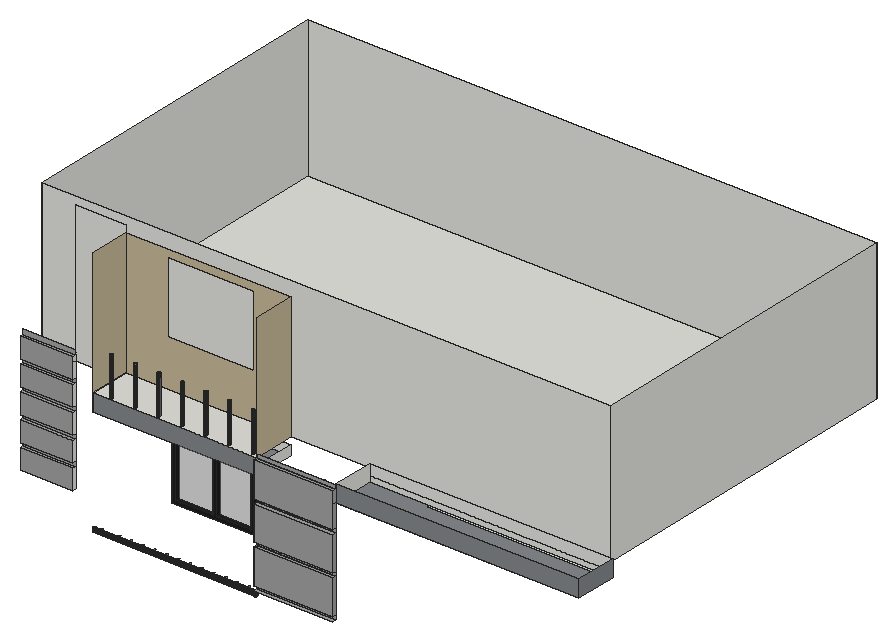
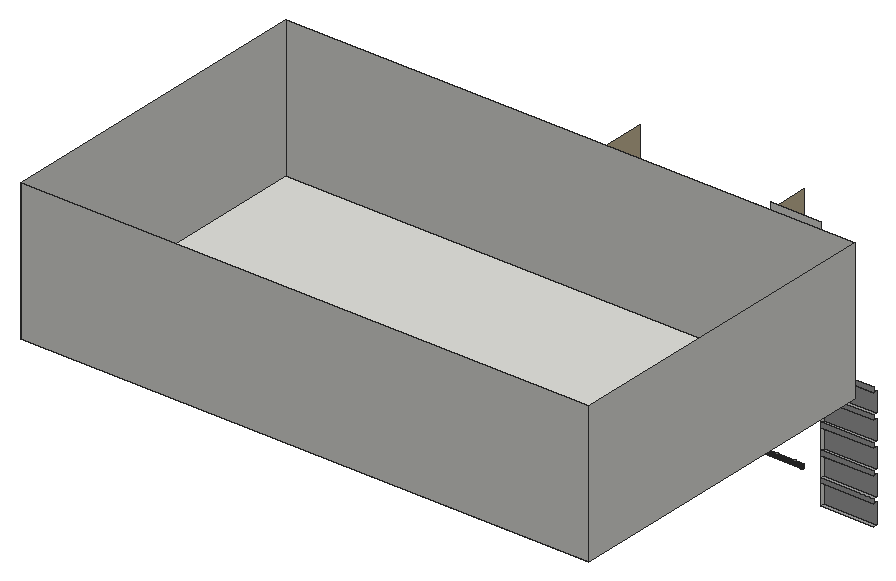
# SketchUp Ruby script. Lengths in inches.
U = 1.inch
M = Sketchup.active_model
def pt(a) = Geom::Point3d.new(a.map { |v| v * U })
def face(e, loops, mat)
  f = e.add_face(loops[0].map { |a| pt(a) })
  loops[1..].each { |l| e.add_face(l.map { |a| pt(a) }).erase! }
  f.material = f.back_material = mat if mat
  f
end
# faces: each face lists its corners as indices into pts; further lists are holes
def faces(e, pts, list, mat = nil) = list.each { |f| face(e, (f[0].is_a?(Array) ? f : [f]).map { |l| l.map { |i| pts[i] } }, mat) }
# xy, xz, yz: faces in a plane at the given z, y or x. An outline is a flat list of corners, or four numbers for a rectangle; further outlines are holes
def ring(l) = l.size == 4 ? [[l[0], l[1]], [l[2], l[1]], [l[2], l[3]], [l[0], l[3]]] : l.each_slice(2).to_a
def flat(e, list, mat, &to3) = list.each { |f| face(e, (f[0].is_a?(Array) ? f : [f]).map { |l| ring(l).map { |u, v| to3.(u, v) } }, mat) }
def xy(e, z, list, mat = nil) = flat(e, list, mat) { |x, y| [x, y, z] }
def xz(e, y, list, mat = nil) = flat(e, list, mat) { |x, z| [x, y, z] }
def yz(e, x, list, mat = nil) = flat(e, list, mat) { |y, z| [x, y, z] }
def lines(e, pts, list) = list.each { |a, b| e.add_line(pt(pts[a]), pt(pts[b])) }
# prism: a flat outline (further loops are holes) pulled along v
def prism(e, loops, v, mat = nil)
  f = face(e, loops, mat); d = Geom::Vector3d.new(v.map { |x| x * U })
  f.pushpull(f.normal.samedirection?(d) ? d.length : -d.length)
end
def box(e, o, s, mat = nil) = prism(e, [[o, [o[0] + s[0], o[1], o[2]], [o[0] + s[0], o[1] + s[1], o[2]], [o[0], o[1] + s[1], o[2]]]], [0, 0, s[2]], mat)
def at(x, y, z, deg = 0) = Geom::Transformation.translation(pt([x, y, z])) * Geom::Transformation.rotation(ORIGIN, Z_AXIS, deg.degrees)
def axes(o, x, y, z) = Geom::Transformation.new([*x, 0, *y, 0, *z, 0, *pt(o).to_a, 1])
def part(name) = M.definitions.add(name)
# library, detail: a bought-in or finely detailed component or shape, given as its bounding box
def library(name, o, s) = part(name).tap { |d| box(d.entities, o, s) }
def detail(e, o, s) = box(e.add_group.entities, o, s)
def put(e, d, t, mat = nil) = e.add_instance(d, t).tap { |i| i.material = mat if mat }
def group(e, t, mat = nil) = e.add_group.tap { |g| g.transformation = t; g.material = mat if mat }.entities
root = M.entities
M.materials.add("[0133_Gray]").color = [128, 128, 128]
M.materials.add("[Blacktop New]").color = [30, 30, 30]
M.materials.add("[Blacktop Old 01]").color = [132, 136, 139]
M.materials.add("[Marble Carrara Gold Floor Tile]").color = [225, 223, 217]
M.materials.add("[Pavers Flagstone Gray]").color = [162, 162, 162]
M.materials.add("[Quartz Light Brown]").color = [199, 184, 152]
M.materials.add("[Translucent Glass Gray]").color = [128, 128, 128]
M.materials["[Translucent Glass Gray]"].alpha = 0.5
xy(root,261.07,[[0,36,45.0625,39]],"[Pavers Flagstone Gray]")
xy(root,263.16,[[95.48,3.83,95.64,3.85,95.79,3.92,95.92,4.02,96.02,4.15,96.08,4.3,96.1,4.46,96.08,4.62,96.02,4.77,95.92,4.9,95.79,5,95.64,5.0625,95.48,5.08,95.32,5.0625,95.17,5,95.04,4.9,94.9375,4.77,94.875,4.62,94.85,4.46,94.875,4.3,94.9375,4.15,95.04,4.02,95.17,3.92,95.32,3.85],[110.48,3.83,110.64,3.85,110.79,3.92,110.92,4.02,111.02,4.15,111.08,4.3,111.1,4.46,111.08,4.62,111.02,4.77,110.92,4.9,110.79,5,110.64,5.0625,110.48,5.08,110.32,5.0625,110.17,5,110.04,4.9,109.9375,4.77,109.875,4.62,109.85,4.46,109.875,4.3,109.9375,4.15,110.04,4.02,110.17,3.92,110.32,3.85],[120.6,3.83,120.77,3.85,120.92,3.92,121.05,4.02,121.15,4.15,121.21,4.3,121.23,4.46,121.21,4.62,121.15,4.77,121.05,4.9,120.92,5,120.77,5.0625,120.6,5.08,120.44,5.0625,120.29,5,120.16,4.9,120.0625,4.77,120,4.62,119.98,4.46,120,4.3,120.0625,4.15,120.16,4.02,120.29,3.92,120.44,3.85],[130.73,3.83,130.89,3.85,131.04,3.92,131.17,4.02,131.27,4.15,131.33,4.3,131.35,4.46,131.33,4.62,131.27,4.77,131.17,4.9,131.04,5,130.89,5.0625,130.73,5.08,130.57,5.0625,130.42,5,130.29,4.9,130.1875,4.77,130.125,4.62,130.1,4.46,130.125,4.3,130.1875,4.15,130.29,4.02,130.42,3.92,130.57,3.85],[140.85,3.83,141.02,3.85,141.17,3.92,141.3,4.02,141.4,4.15,141.46,4.3,141.48,4.46,141.46,4.62,141.4,4.77,141.3,4.9,141.17,5,141.02,5.0625,140.85,5.08,140.69,5.0625,140.54,5,140.41,4.9,140.3125,4.77,140.25,4.62,140.23,4.46,140.25,4.3,140.3125,4.15,140.41,4.02,140.54,3.92,140.69,3.85],
  [150.98,3.83,151.14,3.85,151.29,3.92,151.42,4.02,151.52,4.15,151.58,4.3,151.6,4.46,151.58,4.62,151.52,4.77,151.42,4.9,151.29,5,151.14,5.0625,150.98,5.08,150.82,5.0625,150.67,5,150.54,4.9,150.4375,4.77,150.375,4.62,150.35,4.46,150.375,4.3,150.4375,4.15,150.54,4.02,150.67,3.92,150.82,3.85],[161.1,3.83,161.27,3.85,161.42,3.92,161.55,4.02,161.65,4.15,161.71,4.3,161.73,4.46,161.71,4.62,161.65,4.77,161.55,4.9,161.42,5,161.27,5.0625,161.1,5.08,160.94,5.0625,160.79,5,160.66,4.9,160.5625,4.77,160.5,4.62,160.48,4.46,160.5,4.3,160.5625,4.15,160.66,4.02,160.79,3.92,160.94,3.85],[171.23,3.83,171.39,3.85,171.54,3.92,171.67,4.02,171.77,4.15,171.83,4.3,171.85,4.46,171.83,4.62,171.77,4.77,171.67,4.9,171.54,5,171.39,5.0625,171.23,5.08,171.07,5.0625,170.92,5,170.79,4.9,170.6875,4.77,170.625,4.62,170.6,4.46,170.625,4.3,170.6875,4.15,170.79,4.02,170.92,3.92,171.07,3.85],[181.35,3.83,181.52,3.85,181.67,3.92,181.8,4.02,181.9,4.15,181.96,4.3,181.98,4.46,181.96,4.62,181.9,4.77,181.8,4.9,181.67,5,181.52,5.0625,181.35,5.08,181.19,5.0625,181.04,5,180.91,4.9,180.8125,4.77,180.75,4.62,180.73,4.46,180.75,4.3,180.8125,4.15,180.91,4.02,181.04,3.92,181.19,3.85],[191.48,3.83,191.64,3.85,191.79,3.92,191.92,4.02,192.02,4.15,192.08,4.3,192.1,4.46,192.08,4.62,192.02,4.77,191.92,4.9,191.79,5,191.64,5.0625,191.48,5.08,191.32,5.0625,191.17,5,191.04,4.9,190.9375,4.77,190.875,4.62,190.85,4.46,190.875,4.3,190.9375,4.15,191.04,4.02,191.17,3.92,191.32,3.85],
  [201.6,3.83,201.77,3.85,201.92,3.92,202.05,4.02,202.15,4.15,202.21,4.3,202.23,4.46,202.21,4.62,202.15,4.77,202.05,4.9,201.92,5,201.77,5.0625,201.6,5.08,201.44,5.0625,201.29,5,201.16,4.9,201.0625,4.77,201,4.62,200.98,4.46,201,4.3,201.0625,4.15,201.16,4.02,201.29,3.92,201.44,3.85],[211.73,3.83,211.89,3.85,212.04,3.92,212.17,4.02,212.27,4.15,212.33,4.3,212.35,4.46,212.33,4.62,212.27,4.77,212.17,4.9,212.04,5,211.89,5.0625,211.73,5.08,211.57,5.0625,211.42,5,211.29,4.9,211.1875,4.77,211.125,4.62,211.1,4.46,211.125,4.3,211.1875,4.15,211.29,4.02,211.42,3.92,211.57,3.85],[221.85,3.83,222.02,3.85,222.17,3.92,222.3,4.02,222.4,4.15,222.46,4.3,222.48,4.46,222.46,4.62,222.4,4.77,222.3,4.9,222.17,5,222.02,5.0625,221.85,5.08,221.69,5.0625,221.54,5,221.41,4.9,221.3125,4.77,221.25,4.62,221.23,4.46,221.25,4.3,221.3125,4.15,221.41,4.02,221.54,3.92,221.69,3.85]],"[0133_Gray]")
xy(root,265,[[229.62,0,297.58,3]],"[Pavers Flagstone Gray]")
xy(root,268.62,[[229.62,0,297.58,3]],"[Pavers Flagstone Gray]")
xy(root,278.4375,[[0,36,45.0625,39]],"[Pavers Flagstone Gray]")
xy(root,281.71,[[130.59,36,200.77,39]],"[Blacktop New]")
xy(root,282.51,[[0,36,45.0625,39]],"[Pavers Flagstone Gray]")
xy(root,284.71,[[133.59,36,165.68,39],[168.99,36,197.77,39]],"[Blacktop New]")
xy(root,298.5,[[229.62,0,297.58,3]],"[Pavers Flagstone Gray]")
xy(root,299.875,[[0,36,45.0625,39]],"[Pavers Flagstone Gray]")
xy(root,302.12,[[229.62,0,297.58,3]],"[Pavers Flagstone Gray]")
xy(root,303.95,[[0,36,45.0625,39]],"[Pavers Flagstone Gray]")
xy(root,321.3125,[[0,36,45.0625,39]],"[Pavers Flagstone Gray]")
xy(root,325.39,[[0,36,45.0625,39]],"[Pavers Flagstone Gray]")
xy(root,332,[[229.62,0,297.58,3]],"[Pavers Flagstone Gray]")
xy(root,335.62,[[229.62,0,297.58,3]],"[Pavers Flagstone Gray]")
xy(root,341.28,[[133.59,36,165.68,39],[168.99,36,197.77,39]],"[Blacktop New]")
xy(root,342.75,[[0,36,45.0625,39]],"[Pavers Flagstone Gray]")
xy(root,344.28,[[130.59,36,200.77,39]],"[Blacktop New]")
xy(root,346.82,[[0,36,45.0625,39]],"[Pavers Flagstone Gray]")
xy(root,349.1875,[[355.33,36,420.16,39],[425.68,36,485,39]],"[Blacktop New]")
xy(root,351.5625,[[88.53,3,229.62,39]],"[Blacktop Old 01]")
xy(root,355.1875,[[349.33,36,491,39]])
xy(root,355.1875,[[297.58,3,297.58,39,349.33,39,349.33,36,491,36,491,39,506.625,39,506.625,3]],"[Blacktop Old 01]")
xy(root,360,[[9,48,497.625,333.4375]])
xy(root,364.1875,[[0,36,45.0625,39]],"[Pavers Flagstone Gray]")
xy(root,365.5,[[229.62,0,297.58,3]],"[Pavers Flagstone Gray]")
xy(root,366.04,[[244.21,4.79,244.49,4.8,244.76,4.88,244.99,5.03,245.18,5.23,245.3125,5.48,245.375,5.75,245.36,6.02,245.28,6.29,245.14,6.52,244.93,6.71,244.69,6.84,244.42,6.91,244.14,6.9,243.88,6.82,243.64,6.67,243.45,6.47,243.32,6.22,243.26,5.95,243.27,5.68,243.35,5.41,243.5,5.17,243.7,4.99,243.94,4.85],[264.46,4.79,264.74,4.8,265.01,4.88,265.24,5.03,265.43,5.23,265.5625,5.48,265.625,5.75,265.61,6.02,265.53,6.29,265.39,6.52,265.18,6.71,264.94,6.84,264.67,6.91,264.39,6.9,264.13,6.82,263.89,6.67,263.7,6.47,263.57,6.22,263.51,5.95,263.52,5.68,263.6,5.41,263.75,5.17,263.95,4.99,264.19,4.85],[284.71,4.79,284.99,4.8,285.26,4.88,285.49,5.03,285.68,5.23,285.8125,5.48,285.875,5.75,285.86,6.02,285.78,6.29,285.64,6.52,285.43,6.71,285.19,6.84,284.92,6.91,284.64,6.9,284.38,6.82,284.14,6.67,283.95,6.47,283.82,6.22,283.76,5.95,283.77,5.68,283.85,5.41,284,5.17,284.2,4.99,284.44,4.85],[304.96,4.79,305.24,4.8,305.51,4.88,305.74,5.03,305.93,5.23,306.0625,5.48,306.125,5.75,306.11,6.02,306.03,6.29,305.89,6.52,305.68,6.71,305.44,6.84,305.17,6.91,304.89,6.9,304.63,6.82,304.39,6.67,304.2,6.47,304.07,6.22,304.01,5.95,304.02,5.68,304.1,5.41,304.25,5.17,304.45,4.99,304.69,4.85],[325.21,4.79,325.49,4.8,325.76,4.88,325.99,5.03,326.18,5.23,326.3125,5.48,326.375,5.75,326.36,6.02,326.28,6.29,326.14,6.52,325.93,6.71,325.69,6.84,325.42,6.91,325.14,6.9,324.88,6.82,324.64,6.67,324.45,6.47,324.32,6.22,324.26,5.95,324.27,5.68,324.35,5.41,324.5,5.17,324.7,4.99,324.94,4.85],
  [345.46,4.79,345.74,4.8,346.01,4.88,346.24,5.03,346.43,5.23,346.5625,5.48,346.625,5.75,346.61,6.02,346.53,6.29,346.39,6.52,346.18,6.71,345.94,6.84,345.67,6.91,345.39,6.9,345.13,6.82,344.89,6.67,344.7,6.47,344.57,6.22,344.51,5.95,344.52,5.68,344.6,5.41,344.75,5.17,344.95,4.99,345.19,4.85],[365.71,4.79,365.99,4.8,366.26,4.88,366.49,5.03,366.68,5.23,366.8125,5.48,366.875,5.75,366.86,6.02,366.78,6.29,366.64,6.52,366.43,6.71,366.19,6.84,365.92,6.91,365.64,6.9,365.38,6.82,365.14,6.67,364.95,6.47,364.82,6.22,364.76,5.95,364.77,5.68,364.85,5.41,365,5.17,365.2,4.99,365.44,4.85],[385.96,4.79,386.24,4.8,386.51,4.88,386.74,5.03,386.93,5.23,387.0625,5.48,387.125,5.75,387.11,6.02,387.03,6.29,386.89,6.52,386.68,6.71,386.44,6.84,386.17,6.91,385.89,6.9,385.63,6.82,385.39,6.67,385.2,6.47,385.07,6.22,385.01,5.95,385.02,5.68,385.1,5.41,385.25,5.17,385.45,4.99,385.69,4.85],[406.21,4.79,406.49,4.8,406.76,4.88,406.99,5.03,407.18,5.23,407.3125,5.48,407.375,5.75,407.36,6.02,407.28,6.29,407.14,6.52,406.93,6.71,406.69,6.84,406.42,6.91,406.14,6.9,405.88,6.82,405.64,6.67,405.45,6.47,405.32,6.22,405.26,5.95,405.27,5.68,405.35,5.41,405.5,5.17,405.7,4.99,405.94,4.85]])
xy(root,366.04,[[[88.53,3,229.62,39],[183.46,4.79,183.19,4.85,182.95,4.99,182.75,5.17,182.6,5.41,182.52,5.68,182.51,5.95,182.57,6.22,182.7,6.47,182.89,6.67,183.13,6.82,183.39,6.9,183.67,6.91,183.94,6.84,184.18,6.71,184.39,6.52,184.53,6.29,184.61,6.02,184.625,5.75,184.5625,5.48,184.43,5.23,184.24,5.03,184.01,4.88,183.74,4.8],[203.71,4.79,203.44,4.85,203.2,4.99,203,5.17,202.85,5.41,202.77,5.68,202.76,5.95,202.82,6.22,202.95,6.47,203.14,6.67,203.38,6.82,203.64,6.9,203.92,6.91,204.19,6.84,204.43,6.71,204.64,6.52,204.78,6.29,204.86,6.02,204.875,5.75,204.8125,5.48,204.68,5.23,204.49,5.03,204.26,4.88,203.99,4.8],[223.96,4.79,223.69,4.85,223.45,4.99,223.25,5.17,223.1,5.41,223.02,5.68,223.01,5.95,223.07,6.22,223.2,6.47,223.39,6.67,223.63,6.82,223.89,6.9,224.17,6.91,224.44,6.84,224.68,6.71,224.89,6.52,225.03,6.29,225.11,6.02,225.125,5.75,225.0625,5.48,224.93,5.23,224.74,5.03,224.51,4.88,224.24,4.8],[102.46,4.79,102.19,4.85,101.95,4.99,101.75,5.17,101.6,5.41,101.52,5.68,101.51,5.95,101.57,6.22,101.7,6.47,101.89,6.67,102.13,6.82,102.39,6.9,102.67,6.91,102.94,6.84,103.18,6.71,103.39,6.52,103.53,6.29,103.61,6.02,103.625,5.75,103.5625,5.48,103.43,5.23,103.24,5.03,103.01,4.88,102.74,4.8],[122.71,4.79,122.44,4.85,122.2,4.99,122,5.17,121.85,5.41,121.77,5.68,121.76,5.95,121.82,6.22,121.95,6.47,122.14,6.67,122.38,6.82,122.64,6.9,122.92,6.91,123.19,6.84,123.43,6.71,123.64,6.52,123.78,6.29,123.86,6.02,123.875,5.75,123.8125,5.48,123.68,5.23,123.49,5.03,123.26,4.88,122.99,4.8],[142.96,4.79,142.69,4.85,142.45,4.99,142.25,5.17,142.1,5.41,142.02,5.68,142.01,5.95,142.07,6.22,142.2,6.47,142.39,6.67,142.63,6.82,142.89,6.9,143.17,6.91,143.44,6.84,143.68,6.71,143.89,6.52,144.03,6.29,144.11,6.02,144.125,5.75,144.0625,5.48,143.93,5.23,143.74,5.03,143.51,4.88,143.24,4.8],[163.21,4.79,162.94,4.85,162.7,4.99,162.5,5.17,162.35,5.41,162.27,5.68,162.26,5.95,162.32,6.22,162.45,6.47,162.64,6.67,162.88,6.82,163.14,6.9,163.42,6.91,163.69,6.84,163.93,6.71,164.14,6.52,164.28,6.29,164.36,6.02,164.375,5.75,164.3125,5.48,164.18,5.23,163.99,5.03,163.76,4.88,163.49,4.8]]],"[Marble Carrara Gold Floor Tile]")
xz(root,0,[[229.62,268.62,297.58,298.5],[229.62,302.12,297.58,332],[229.62,335.62,297.58,365.5]],"[Pavers Flagstone Gray]")
xz(root,3,[[229.62,268.62,297.58,298.5],[229.62,302.12,297.58,332],[229.62,335.62,297.58,365.5]])
xz(root,3,[[88.53,351.5625,229.62,366.04],[297.58,355.1875,506.625,369.51]],"[Blacktop Old 01]")
xz(root,3,[[229.62,265,297.58,268.62],[229.62,298.5,297.58,302.12],[229.62,332,297.58,335.62],[229.62,365.5,297.58,369.12]],"[Pavers Flagstone Gray]")
xz(root,36,[[[130.59,281.71,200.77,344.28],[133.59,284.71,165.68,341.28],[168.99,284.71,197.77,341.28]]],"[Blacktop New]")
xz(root,36,[[0,261.07,45.0625,278.4375],[0,282.51,45.0625,299.875],[0,303.95,45.0625,321.3125],[0,325.39,45.0625,342.75],[0,346.82,45.0625,364.1875]],"[Pavers Flagstone Gray]")
xz(root,39,[[88.53,351.5625,229.62,359.8125],[297.58,355.1875,506.625,359.8125],[88.53,359.8125,229.62,360],[297.58,359.8125,506.625,369.51],[45.0625,360,88.53,480]])
xz(root,39,[[0,278.4375,45.0625,282.51],[0,299.875,45.0625,303.95],[0,321.3125,45.0625,325.39],[0,342.75,45.0625,346.82],[0,364.1875,45.0625,368.26]],"[Pavers Flagstone Gray]")
xz(root,39,[[[88.53,366.04,229.62,473.6875],[124.42,405.86,198.67,467.74]]],"[Quartz Light Brown]")
xz(root,39,[[133.59,284.71,165.68,341.28],[168.99,284.71,197.77,341.28]],"[Translucent Glass Gray]")
xz(root,48,[[9,360,497.625,480]])
xz(root,333.4375,[[9,360,497.625,480]])
yz(root,9,[[48,360,333.4375,480]])
yz(root,45.0625,[[36,261.07,39,278.4375],[36,282.51,39,299.875],[36,303.95,39,321.3125],[36,325.39,39,342.75],[36,346.82,39,360],
  [36,360,39,364.1875]])
yz(root,88.53,[[3,351.5625,39,360],[3,360,39,366.04]])
yz(root,88.53,[[[3,366.04,39,473.6875],[3.75,370.61,3.57,370.63,3.41,370.7,3.27,370.81,3.16,370.95,3.09,371.11,3.06,371.29,3.09,371.47,3.16,371.64,3.27,371.78,3.41,371.89,3.57,371.96,3.75,371.98,3.93,371.96,4.1,371.89,4.24,371.78,4.35,371.64,4.42,371.47,4.44,371.29,4.42,371.11,4.35,370.95,4.24,370.81,4.1,370.7,3.93,370.63],[3.75,374.36,3.57,374.38,3.41,374.45,3.27,374.56,3.16,374.7,3.09,374.86,3.06,375.04,3.09,375.22,3.16,375.39,3.27,375.53,3.41,375.64,3.57,375.71,3.75,375.73,3.93,375.71,4.1,375.64,4.24,375.53,4.35,375.39,4.42,375.22,4.44,375.04,4.42,374.86,4.35,374.7,4.24,374.56,4.1,374.45,3.93,374.38],[3.75,378.11,3.57,378.13,3.41,378.2,3.27,378.31,3.16,378.45,3.09,378.61,3.06,378.79,3.09,378.97,3.16,379.14,3.27,379.28,3.41,379.39,3.57,379.46,3.75,379.48,3.93,379.46,4.1,379.39,4.24,379.28,4.35,379.14,4.42,378.97,4.44,378.79,4.42,378.61,4.35,378.45,4.24,378.31,4.1,378.2,3.93,378.13],[3.75,381.86,3.57,381.88,3.41,381.95,3.27,382.06,3.16,382.2,3.09,382.36,3.06,382.54,3.09,382.72,3.16,382.89,3.27,383.03,3.41,383.14,3.57,383.21,3.75,383.23,3.93,383.21,4.1,383.14,4.24,383.03,4.35,382.89,4.42,382.72,4.44,382.54,4.42,382.36,4.35,382.2,4.24,382.06,4.1,381.95,3.93,381.88],[3.75,385.61,3.57,385.63,3.41,385.7,3.27,385.81,3.16,385.95,3.09,386.11,3.06,386.29,3.09,386.47,3.16,386.64,3.27,386.78,3.41,386.89,3.57,386.96,3.75,386.98,3.93,386.96,4.1,386.89,4.24,386.78,4.35,386.64,4.42,386.47,4.44,386.29,4.42,386.11,4.35,385.95,4.24,385.81,4.1,385.7,3.93,385.63],[3.75,389.36,3.57,389.38,3.41,389.45,3.27,389.56,3.16,389.7,3.09,389.86,3.06,390.04,3.09,390.22,3.16,390.39,3.27,390.53,3.41,390.64,3.57,390.71,3.75,390.73,3.93,390.71,4.1,390.64,4.24,390.53,4.35,390.39,4.42,390.22,4.44,390.04,4.42,389.86,4.35,389.7,4.24,389.56,4.1,389.45,3.93,389.38],[3.75,393.11,3.57,393.13,3.41,393.2,3.27,393.31,3.16,393.45,3.09,393.61,3.06,393.79,3.09,393.97,3.16,394.14,3.27,394.28,3.41,394.39,3.57,394.46,3.75,394.48,3.93,394.46,4.1,394.39,4.24,394.28,4.35,394.14,4.42,393.97,4.44,393.79,4.42,393.61,4.35,393.45,4.24,393.31,4.1,393.2,3.93,393.13],[3.75,396.86,3.57,396.88,3.41,396.95,3.27,397.06,3.16,397.2,3.09,397.36,3.06,397.54,3.09,397.72,3.16,397.89,3.27,398.03,3.41,398.14,3.57,398.21,3.75,398.23,3.93,398.21,4.1,398.14,4.24,398.03,4.35,397.89,4.42,397.72,4.44,397.54,4.42,397.36,4.35,397.2,4.24,397.06,4.1,396.95,3.93,396.88]]],"[Quartz Light Brown]")
yz(root,130.59,[[36,281.71,39,344.28]],"[Blacktop New]")
yz(root,133.59,[[36,284.71,39,341.28]],"[Blacktop New]")
yz(root,165.68,[[36,284.71,39,341.28]],"[Blacktop New]")
yz(root,168.99,[[36,284.71,39,341.28]],"[Blacktop New]")
yz(root,197.77,[[36,284.71,39,341.28]],"[Blacktop New]")
yz(root,200.77,[[36,281.71,39,344.28]],"[Blacktop New]")
yz(root,229.62,[[3,351.5625,39,360]])
yz(root,229.62,[[0,268.62,3,298.5],[0,302.12,3,332],[0,335.62,3,365.5]],"[Pavers Flagstone Gray]")
yz(root,229.62,[[[3,366.04,39,473.6875],[3.75,389.36,3.93,389.38,4.1,389.45,4.24,389.56,4.35,389.7,4.42,389.86,4.44,390.04,4.42,390.22,4.35,390.39,4.24,390.53,4.1,390.64,3.93,390.71,3.75,390.73,3.57,390.71,3.41,390.64,3.27,390.53,3.16,390.39,3.09,390.22,3.06,390.04,3.09,389.86,3.16,389.7,3.27,389.56,3.41,389.45,3.57,389.38],[3.75,385.61,3.93,385.63,4.1,385.7,4.24,385.81,4.35,385.95,4.42,386.11,4.44,386.29,4.42,386.47,4.35,386.64,4.24,386.78,4.1,386.89,3.93,386.96,3.75,386.98,3.57,386.96,3.41,386.89,3.27,386.78,3.16,386.64,3.09,386.47,3.06,386.29,3.09,386.11,3.16,385.95,3.27,385.81,3.41,385.7,3.57,385.63],[3.75,381.86,3.93,381.88,4.1,381.95,4.24,382.06,4.35,382.2,4.42,382.36,4.44,382.54,4.42,382.72,4.35,382.89,4.24,383.03,4.1,383.14,3.93,383.21,3.75,383.23,3.57,383.21,3.41,383.14,3.27,383.03,3.16,382.89,3.09,382.72,3.06,382.54,3.09,382.36,3.16,382.2,3.27,382.06,3.41,381.95,3.57,381.88],[3.75,378.11,3.93,378.13,4.1,378.2,4.24,378.31,4.35,378.45,4.42,378.61,4.44,378.79,4.42,378.97,4.35,379.14,4.24,379.28,4.1,379.39,3.93,379.46,3.75,379.48,3.57,379.46,3.41,379.39,3.27,379.28,3.16,379.14,3.09,378.97,3.06,378.79,3.09,378.61,3.16,378.45,3.27,378.31,3.41,378.2,3.57,378.13]]],"[Quartz Light Brown]")
yz(root,297.58,[[3,355.1875,39,369.51]])
yz(root,297.58,[[0,268.62,3,298.5],[0,302.12,3,332],[0,335.62,3,355.1875],[0,355.1875,3,365.5]],"[Pavers Flagstone Gray]")
yz(root,497.625,[[48,360,333.4375,480]])
yz(root,506.625,[[3,355.1875,39,369.51]],"[Blacktop Old 01]")
p = [[88.53,3.34,258.9375],[88.53,3.43,258.9],[229.62,3.43,258.9],[229.62,3.34,258.9375],[88.53,3.26,259],[229.62,3.26,259],
  [88.53,3.53,258.89],[229.62,3.53,258.89],[88.53,3.625,258.9],[229.62,3.625,258.9],[88.53,3.71,258.9375],[229.62,3.71,258.9375],
  [88.53,3.79,259],[229.62,3.79,259],[88.53,3.2,259.08],[229.62,3.2,259.08],[88.53,3.85,259.08],[229.62,3.85,259.08],
  [88.53,3.16,259.17],[229.62,3.16,259.17],[88.53,3.89,259.17],[229.62,3.89,259.17],[88.53,3.15,259.26],[229.62,3.15,259.26],
  [88.53,3.9,259.26],[229.62,3.9,259.26],[88.53,3.16,259.36],[229.62,3.16,259.36],[88.53,3.89,259.36],[229.62,3.89,259.36],
  [88.53,3.2,259.45],[229.62,3.2,259.45],[88.53,3.85,259.45],[229.62,3.85,259.45],[88.53,3.26,259.53],[229.62,3.26,259.53],
  [88.53,3.34,259.59],[229.62,3.34,259.59],[88.53,3.79,259.53],[88.53,3.71,259.59],[229.62,3.71,259.59],[229.62,3.79,259.53],
  [88.53,3.43,259.625],[229.62,3.43,259.625],[88.53,3.53,259.64],[229.62,3.53,259.64],[88.53,3.625,259.625],[229.62,3.625,259.625],
  [88.53,3.34,260.5],[88.53,3.43,260.46],[229.62,3.43,260.46],[229.62,3.34,260.5],[88.53,3.26,260.56],[229.62,3.26,260.56],
  [88.53,3.53,260.45],[229.62,3.53,260.45],[88.53,3.625,260.46],[229.62,3.625,260.46],[88.53,3.71,260.5],[229.62,3.71,260.5],
  [88.53,3.79,260.56],[229.62,3.79,260.56],[88.53,3.2,260.64],[229.62,3.2,260.64],[88.53,3.16,260.73],[229.62,3.16,260.73],
  [88.53,3.85,260.64],[229.62,3.85,260.64],[88.53,3.89,260.73],[229.62,3.89,260.73],[88.53,3.15,260.83],[229.62,3.15,260.83],
  [88.53,3.9,260.83],[229.62,3.9,260.83],[88.53,3.16,260.92],[229.62,3.16,260.92],[88.53,3.89,260.92],[229.62,3.89,260.92],
  [88.53,3.2,261.01],[229.62,3.2,261.01],[88.53,3.85,261.01],[229.62,3.85,261.01],[88.53,3.26,261.09],[229.62,3.26,261.09],
  [88.53,3.79,261.09],[229.62,3.79,261.09],[88.53,3.34,261.15],[229.62,3.34,261.15],[88.53,3.43,261.1875],[229.62,3.43,261.1875],
  [88.53,3.71,261.15],[88.53,3.625,261.1875],[229.62,3.625,261.1875],[229.62,3.71,261.15],[88.53,3.53,261.2],[229.62,3.53,261.2],
  [88.53,3.34,262.0625],[88.53,3.43,262.03],[229.62,3.43,262.03],[229.62,3.34,262.0625],[88.53,3.53,262.01],[229.62,3.53,262.01],
  [88.53,3.625,262.03],[229.62,3.625,262.03],[88.53,3.71,262.0625],[229.62,3.71,262.0625],[88.53,3.2,262.2],[88.53,3.26,262.12],
  [229.62,3.26,262.12],[229.62,3.2,262.2],[88.53,3.79,262.12],[229.62,3.79,262.12],[88.53,3.85,262.2],[229.62,3.85,262.2],
  [88.53,3.16,262.29],[229.62,3.16,262.29],[88.53,3.89,262.29],[229.62,3.89,262.29],[88.53,3.15,262.39],[229.62,3.15,262.39],
  [88.53,3.9,262.39],[229.62,3.9,262.39],[88.53,3.16,262.48],[229.62,3.16,262.48],[88.53,3.89,262.48],[229.62,3.89,262.48],
  [88.53,3.2,262.58],[229.62,3.2,262.58],[88.53,3.85,262.58],[229.62,3.85,262.58],[88.53,3.26,262.65],[229.62,3.26,262.65],
  [88.53,3.79,262.65],[229.62,3.79,262.65],[88.53,3.34,262.71],[229.62,3.34,262.71],[88.53,3.43,262.75],[229.62,3.43,262.75],
  [88.53,3.53,262.76],[229.62,3.53,262.76],[88.53,3.625,262.75],[229.62,3.625,262.75],[88.53,3.71,262.71],[229.62,3.71,262.71],
  [102.19,4.85,366.04],[102.46,4.79,366.04],[102.46,4.79,399.54],[102.19,4.85,399.54],[102.74,4.8,366.04],[102.74,4.8,399.54],
  [103.01,4.88,366.04],[103.01,4.88,399.54],[122.44,4.85,366.04],[122.71,4.79,366.04],[122.71,4.79,399.54],[122.44,4.85,399.54],
  [122.99,4.8,366.04],[122.99,4.8,399.54],[123.26,4.88,366.04],[123.26,4.88,399.54],[142.69,4.85,366.04],[142.96,4.79,366.04],
  [142.96,4.79,399.54],[142.69,4.85,399.54],[143.24,4.8,366.04],[143.24,4.8,399.54],[143.51,4.88,366.04],[143.51,4.88,399.54],
  [162.94,4.85,366.04],[163.21,4.79,366.04],[163.21,4.79,399.54],[162.94,4.85,399.54],[163.49,4.8,366.04],[163.49,4.8,399.54],
  [163.76,4.88,366.04],[163.76,4.88,399.54],[183.19,4.85,366.04],[183.46,4.79,366.04],[183.46,4.79,399.54],[183.19,4.85,399.54],
  [183.74,4.8,366.04],[183.74,4.8,399.54],[184.01,4.88,366.04],[184.01,4.88,399.54],[203.44,4.85,366.04],[203.71,4.79,366.04],
  [203.71,4.79,399.54],[203.44,4.85,399.54],[203.99,4.8,366.04],[203.99,4.8,399.54],[204.26,4.88,366.04],[204.26,4.88,399.54],
  [223.69,4.85,366.04],[223.96,4.79,366.04],[223.96,4.79,399.54],[223.69,4.85,399.54],[224.24,4.8,366.04],[224.24,4.8,399.54],
  [224.51,4.88,366.04],[224.51,4.88,399.54],[101.95,4.99,366.04],[101.95,4.99,399.54],[103.24,5.03,366.04],[103.24,5.03,399.54],
  [122.2,4.99,366.04],[122.2,4.99,399.54],[123.49,5.03,366.04],[123.49,5.03,399.54],[142.45,4.99,366.04],[142.45,4.99,399.54],
  [143.74,5.03,366.04],[143.74,5.03,399.54],[162.7,4.99,366.04],[162.7,4.99,399.54],[163.99,5.03,366.04],[163.99,5.03,399.54],
  [182.95,4.99,366.04],[182.95,4.99,399.54],[184.24,5.03,366.04],[184.24,5.03,399.54],[203.2,4.99,366.04],[203.2,4.99,399.54],
  [204.49,5.03,366.04],[204.49,5.03,399.54],[223.45,4.99,366.04],[223.45,4.99,399.54],[224.74,5.03,366.04],[224.74,5.03,399.54],
  [101.75,5.17,366.04],[101.75,5.17,399.54],[103.43,5.23,366.04],[103.43,5.23,399.54],[122,5.17,366.04],[122,5.17,399.54],
  [123.68,5.23,366.04],[123.68,5.23,399.54],[142.25,5.17,366.04],[142.25,5.17,399.54],[143.93,5.23,366.04],[143.93,5.23,399.54],
  [162.5,5.17,366.04],[162.5,5.17,399.54],[164.18,5.23,366.04],[164.18,5.23,399.54],[182.75,5.17,366.04],[182.75,5.17,399.54],
  [184.43,5.23,366.04],[184.43,5.23,399.54],[203,5.17,366.04],[203,5.17,399.54],[204.68,5.23,366.04],[204.68,5.23,399.54],
  [223.25,5.17,366.04],[223.25,5.17,399.54],[224.93,5.23,366.04],[224.93,5.23,399.54],[101.6,5.41,366.04],[101.6,5.41,399.54],
  [103.5625,5.48,366.04],[103.5625,5.48,399.54],[121.85,5.41,366.04],[121.85,5.41,399.54],[123.8125,5.48,366.04],[123.8125,5.48,399.54],
  [142.1,5.41,366.04],[142.1,5.41,399.54],[144.0625,5.48,366.04],[144.0625,5.48,399.54],[162.35,5.41,366.04],[162.35,5.41,399.54],
  [164.3125,5.48,366.04],[164.3125,5.48,399.54],[182.6,5.41,366.04],[182.6,5.41,399.54],[184.5625,5.48,366.04],[184.5625,5.48,399.54],
  [202.85,5.41,366.04],[202.85,5.41,399.54],[204.8125,5.48,366.04],[204.8125,5.48,399.54],[223.1,5.41,366.04],[223.1,5.41,399.54],
  [225.0625,5.48,366.04],[225.0625,5.48,399.54],[101.52,5.68,366.04],[101.52,5.68,399.54],[121.77,5.68,366.04],[121.77,5.68,399.54],
  [142.02,5.68,366.04],[142.02,5.68,399.54],[162.27,5.68,366.04],[162.27,5.68,399.54],[182.52,5.68,366.04],[182.52,5.68,399.54],
  [202.77,5.68,366.04],[202.77,5.68,399.54],[223.02,5.68,366.04],[223.02,5.68,399.54],[103.625,5.75,366.04],[103.625,5.75,399.54],
  [123.875,5.75,366.04],[123.875,5.75,399.54],[144.125,5.75,366.04],[144.125,5.75,399.54],[164.375,5.75,366.04],[164.375,5.75,399.54],
  [184.625,5.75,366.04],[184.625,5.75,399.54],[204.875,5.75,366.04],[204.875,5.75,399.54],[225.125,5.75,366.04],[225.125,5.75,399.54],
  [101.51,5.95,366.04],[101.51,5.95,399.54],[103.61,6.02,366.04],[103.61,6.02,399.54],[121.76,5.95,366.04],[121.76,5.95,399.54],
  [123.86,6.02,366.04],[123.86,6.02,399.54],[142.01,5.95,366.04],[142.01,5.95,399.54],[144.11,6.02,366.04],[144.11,6.02,399.54],
  [162.26,5.95,366.04],[162.26,5.95,399.54],[164.36,6.02,366.04],[164.36,6.02,399.54],[182.51,5.95,366.04],[182.51,5.95,399.54],
  [184.61,6.02,366.04],[184.61,6.02,399.54],[202.76,5.95,366.04],[202.76,5.95,399.54],[204.86,6.02,366.04],[204.86,6.02,399.54],
  [223.01,5.95,366.04],[223.01,5.95,399.54],[225.11,6.02,366.04],[225.11,6.02,399.54],[101.57,6.22,366.04],[101.57,6.22,399.54],
  [103.53,6.29,366.04],[103.53,6.29,399.54],[121.82,6.22,366.04],[121.82,6.22,399.54],[123.78,6.29,366.04],[123.78,6.29,399.54],
  [142.07,6.22,366.04],[142.07,6.22,399.54],[144.03,6.29,366.04],[144.03,6.29,399.54],[162.32,6.22,366.04],[162.32,6.22,399.54],
  [164.28,6.29,366.04],[164.28,6.29,399.54],[182.57,6.22,366.04],[182.57,6.22,399.54],[184.53,6.29,366.04],[184.53,6.29,399.54],
  [202.82,6.22,366.04],[202.82,6.22,399.54],[204.78,6.29,366.04],[204.78,6.29,399.54],[223.07,6.22,366.04],[223.07,6.22,399.54],
  [225.03,6.29,366.04],[225.03,6.29,399.54],[101.7,6.47,366.04],[101.7,6.47,399.54],[121.95,6.47,366.04],[121.95,6.47,399.54],
  [142.2,6.47,366.04],[142.2,6.47,399.54],[162.45,6.47,366.04],[162.45,6.47,399.54],[182.7,6.47,366.04],[182.7,6.47,399.54],
  [202.95,6.47,366.04],[202.95,6.47,399.54],[223.2,6.47,366.04],[223.2,6.47,399.54],[103.39,6.52,366.04],[103.39,6.52,399.54],
  [123.64,6.52,366.04],[123.64,6.52,399.54],[143.89,6.52,366.04],[143.89,6.52,399.54],[164.14,6.52,366.04],[164.14,6.52,399.54],
  [184.39,6.52,366.04],[184.39,6.52,399.54],[204.64,6.52,366.04],[204.64,6.52,399.54],[224.89,6.52,366.04],[224.89,6.52,399.54],
  [101.89,6.67,366.04],[101.89,6.67,399.54],[103.18,6.71,366.04],[103.18,6.71,399.54],[122.14,6.67,366.04],[122.14,6.67,399.54],
  [123.43,6.71,366.04],[123.43,6.71,399.54],[142.39,6.67,366.04],[142.39,6.67,399.54],[143.68,6.71,366.04],[143.68,6.71,399.54],
  [162.64,6.67,366.04],[162.64,6.67,399.54],[163.93,6.71,366.04],[163.93,6.71,399.54],[182.89,6.67,366.04],[182.89,6.67,399.54],
  [184.18,6.71,366.04],[184.18,6.71,399.54],[203.14,6.67,366.04],[203.14,6.67,399.54],[204.43,6.71,366.04],[204.43,6.71,399.54],
  [223.39,6.67,366.04],[223.39,6.67,399.54],[224.68,6.71,366.04],[224.68,6.71,399.54],[102.13,6.82,366.04],[102.13,6.82,399.54],
  [102.94,6.84,366.04],[102.94,6.84,399.54],[122.38,6.82,366.04],[122.38,6.82,399.54],[123.19,6.84,366.04],[123.19,6.84,399.54],
  [142.63,6.82,366.04],[142.63,6.82,399.54],[143.44,6.84,366.04],[143.44,6.84,399.54],[162.88,6.82,366.04],[162.88,6.82,399.54],
  [163.69,6.84,366.04],[163.69,6.84,399.54],[183.13,6.82,366.04],[183.13,6.82,399.54],[183.94,6.84,366.04],[183.94,6.84,399.54],
  [203.38,6.82,366.04],[203.38,6.82,399.54],[204.19,6.84,366.04],[204.19,6.84,399.54],[223.63,6.82,366.04],[223.63,6.82,399.54],
  [224.44,6.84,366.04],[224.44,6.84,399.54],[102.39,6.9,366.04],[102.39,6.9,399.54],[102.67,6.91,366.04],[102.67,6.91,399.54],
  [122.64,6.9,366.04],[122.64,6.9,399.54],[122.92,6.91,366.04],[122.92,6.91,399.54],[142.89,6.9,366.04],[142.89,6.9,399.54],
  [143.17,6.91,366.04],[143.17,6.91,399.54],[163.14,6.9,366.04],[163.14,6.9,399.54],[163.42,6.91,366.04],[163.42,6.91,399.54],
  [183.39,6.9,366.04],[183.39,6.9,399.54],[183.67,6.91,366.04],[183.67,6.91,399.54],[203.64,6.9,366.04],[203.64,6.9,399.54],
  [203.92,6.91,366.04],[203.92,6.91,399.54],[223.89,6.9,366.04],[223.89,6.9,399.54],[224.17,6.91,366.04],[224.17,6.91,399.54]]
faces(root,p,[[0,1,2,3],[4,0,3,5],[1,6,7,2],[6,8,9,7],[8,10,11,9],[10,12,13,11],[14,4,5,15],[12,16,17,13],
  [18,14,15,19],[16,20,21,17],[22,18,19,23],[20,24,25,21],[26,22,23,27],[24,28,29,25],[30,26,27,31],[28,32,33,29],
  [34,30,31,35],[36,34,35,37],[38,39,40,41],[32,38,41,33],[42,36,37,43],[44,42,43,45],[46,44,45,47],[39,46,47,40],
  [48,49,50,51],[52,48,51,53],[49,54,55,50],[54,56,57,55],[56,58,59,57],[58,60,61,59],[62,52,53,63],[64,62,63,65],
  [60,66,67,61],[66,68,69,67],[70,64,65,71],[68,72,73,69],[74,70,71,75],[72,76,77,73],[78,74,75,79],[76,80,81,77],
  [82,78,79,83],[80,84,85,81],[86,82,83,87],[88,86,87,89],[90,91,92,93],[84,90,93,85],[94,88,89,95],[91,94,95,92],
  [96,97,98,99],[97,100,101,98],[100,102,103,101],[102,104,105,103],[106,107,108,109],[107,96,99,108],[104,110,111,105],[110,112,113,111],
  [114,106,109,115],[112,116,117,113],[118,114,115,119],[116,120,121,117],[122,118,119,123],[120,124,125,121],[126,122,123,127],[124,128,129,125],
  [130,126,127,131],[128,132,133,129],[134,130,131,135],[136,134,135,137],[138,136,137,139],[140,138,139,141],[142,140,141,143],[132,142,143,133],
  [144,145,146,147],[145,148,149,146],[148,150,151,149],[152,153,154,155],[153,156,157,154],[156,158,159,157],[160,161,162,163],[161,164,165,162],
  [164,166,167,165],[168,169,170,171],[169,172,173,170],[172,174,175,173],[176,177,178,179],[177,180,181,178],[180,182,183,181],[184,185,186,187],
  [185,188,189,186],[188,190,191,189],[192,193,194,195],[193,196,197,194],[196,198,199,197],[200,144,147,201],[150,202,203,151],[204,152,155,205],
  [158,206,207,159],[208,160,163,209],[166,210,211,167],[212,168,171,213],[174,214,215,175],[216,176,179,217],[182,218,219,183],[220,184,187,221],
  [190,222,223,191],[224,192,195,225],[198,226,227,199],[228,200,201,229],[202,230,231,203],[232,204,205,233],[206,234,235,207],[236,208,209,237],
  [210,238,239,211],[240,212,213,241],[214,242,243,215],[244,216,217,245],[218,246,247,219],[248,220,221,249],[222,250,251,223],[252,224,225,253],
  [226,254,255,227],[256,228,229,257],[230,258,259,231],[260,232,233,261],[234,262,263,235],[264,236,237,265],[238,266,267,239],[268,240,241,269],
  [242,270,271,243],[272,244,245,273],[246,274,275,247],[276,248,249,277],[250,278,279,251],[280,252,253,281],[254,282,283,255],[284,256,257,285],
  [286,260,261,287],[288,264,265,289],[290,268,269,291],[292,272,273,293],[294,276,277,295],[296,280,281,297],[258,298,299,259],[262,300,301,263],
  [266,302,303,267],[270,304,305,271],[274,306,307,275],[278,308,309,279],[282,310,311,283],[312,284,285,313],[298,314,315,299],[316,286,287,317],
  [300,318,319,301],[320,288,289,321],[302,322,323,303],[324,290,291,325],[304,326,327,305],[328,292,293,329],[306,330,331,307],[332,294,295,333],
  [308,334,335,309],[336,296,297,337],[310,338,339,311],[340,312,313,341],[314,342,343,315],[344,316,317,345],[318,346,347,319],[348,320,321,349],
  [322,350,351,323],[352,324,325,353],[326,354,355,327],[356,328,329,357],[330,358,359,331],[360,332,333,361],[334,362,363,335],[364,336,337,365],
  [338,366,367,339],[368,340,341,369],[370,344,345,371],[372,348,349,373],[374,352,353,375],[376,356,357,377],[378,360,361,379],[380,364,365,381],
  [342,382,383,343],[346,384,385,347],[350,386,387,351],[354,388,389,355],[358,390,391,359],[362,392,393,363],[366,394,395,367],[396,368,369,397],
  [382,398,399,383],[400,370,371,401],[384,402,403,385],[404,372,373,405],[386,406,407,387],[408,374,375,409],[388,410,411,389],[412,376,377,413],
  [390,414,415,391],[416,378,379,417],[392,418,419,393],[420,380,381,421],[394,422,423,395],[424,396,397,425],[398,426,427,399],[428,400,401,429],
  [402,430,431,403],[432,404,405,433],[406,434,435,407],[436,408,409,437],[410,438,439,411],[440,412,413,441],[414,442,443,415],[444,416,417,445],
  [418,446,447,419],[448,420,421,449],[422,450,451,423],[452,424,425,453],[426,454,455,427],[456,428,429,457],[430,458,459,431],[460,432,433,461],
  [434,462,463,435],[464,436,437,465],[438,466,467,439],[468,440,441,469],[442,470,471,443],[472,444,445,473],[446,474,475,447],[476,448,449,477],
  [450,478,479,451],[454,452,453,455],[458,456,457,459],[462,460,461,463],[466,464,465,467],[470,468,469,471],[474,472,473,475],[478,476,477,479]],"[0133_Gray]")
